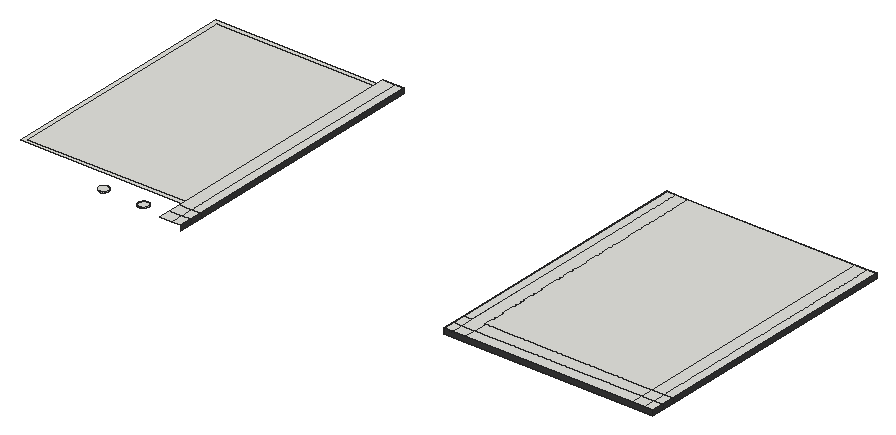
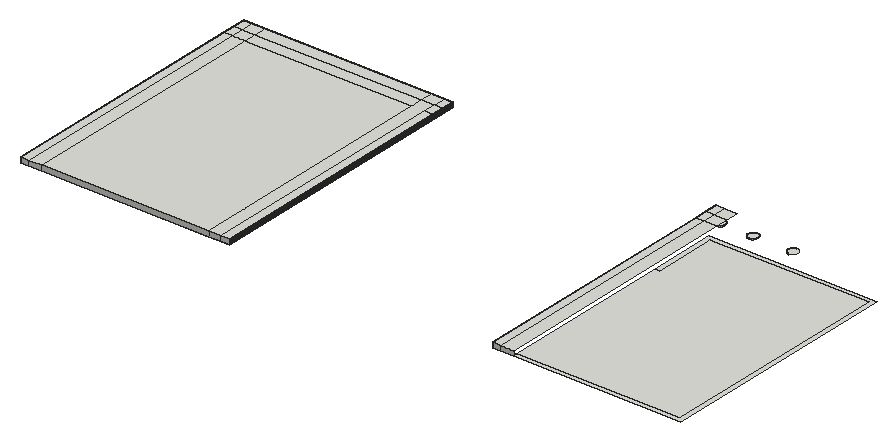
# SketchUp Ruby script. Lengths in inches.
U = 1.inch
M = Sketchup.active_model
def pt(a) = Geom::Point3d.new(a.map { |v| v * U })
def face(e, loops, mat)
  f = e.add_face(loops[0].map { |a| pt(a) })
  loops[1..].each { |l| e.add_face(l.map { |a| pt(a) }).erase! }
  f.material = f.back_material = mat if mat
  f
end
# faces: each face lists its corners as indices into pts; further lists are holes
def faces(e, pts, list, mat = nil) = list.each { |f| face(e, (f[0].is_a?(Array) ? f : [f]).map { |l| l.map { |i| pts[i] } }, mat) }
# xy, xz, yz: faces in a plane at the given z, y or x. An outline is a flat list of corners, or four numbers for a rectangle; further outlines are holes
def ring(l) = l.size == 4 ? [[l[0], l[1]], [l[2], l[1]], [l[2], l[3]], [l[0], l[3]]] : l.each_slice(2).to_a
def flat(e, list, mat, &to3) = list.each { |f| face(e, (f[0].is_a?(Array) ? f : [f]).map { |l| ring(l).map { |u, v| to3.(u, v) } }, mat) }
def xy(e, z, list, mat = nil) = flat(e, list, mat) { |x, y| [x, y, z] }
def xz(e, y, list, mat = nil) = flat(e, list, mat) { |x, z| [x, y, z] }
def yz(e, x, list, mat = nil) = flat(e, list, mat) { |y, z| [x, y, z] }
def lines(e, pts, list) = list.each { |a, b| e.add_line(pt(pts[a]), pt(pts[b])) }
# prism: a flat outline (further loops are holes) pulled along v
def prism(e, loops, v, mat = nil)
  f = face(e, loops, mat); d = Geom::Vector3d.new(v.map { |x| x * U })
  f.pushpull(f.normal.samedirection?(d) ? d.length : -d.length)
end
def box(e, o, s, mat = nil) = prism(e, [[o, [o[0] + s[0], o[1], o[2]], [o[0] + s[0], o[1] + s[1], o[2]], [o[0], o[1] + s[1], o[2]]]], [0, 0, s[2]], mat)
def at(x, y, z, deg = 0) = Geom::Transformation.translation(pt([x, y, z])) * Geom::Transformation.rotation(ORIGIN, Z_AXIS, deg.degrees)
def axes(o, x, y, z) = Geom::Transformation.new([*x, 0, *y, 0, *z, 0, *pt(o).to_a, 1])
def part(name) = M.definitions.add(name)
# library, detail: a bought-in or finely detailed component or shape, given as its bounding box
def library(name, o, s) = part(name).tap { |d| box(d.entities, o, s) }
def detail(e, o, s) = box(e.add_group.entities, o, s)
def put(e, d, t, mat = nil) = e.add_instance(d, t).tap { |i| i.material = mat if mat }
def group(e, t, mat = nil) = e.add_group.tap { |g| g.transformation = t; g.material = mat if mat }.entities
root = M.entities
M.materials.add("[Color C08]").color = [58, 29, 0]
M.materials.add("[Color M07]").color = [58, 58, 58]
xy(root,502.5625,[[649.1875,283.04,848.4,283.04,848.4,362.98,843.96,362.98,843.96,287.65,653.8,287.65,653.8,570.3125,848.4,570.3125,848.4,574.92,649.1875,574.92],[1212.3125,283.04,1411.53,283.04,1411.53,362.98,1407.08,362.98,1407.08,287.65,1216.92,287.65,1216.92,570.3125,1411.53,570.3125,1411.53,574.92,1212.3125,574.92],[653.8,287.65,653.8,570.3125,848.4,570.3125,848.4,362.98,843.96,362.98,843.96,287.65],[1216.92,287.65,1216.92,570.3125,1411.53,570.3125,1411.53,362.98,1407.08,362.98,1407.08,287.65],[848.4,570.3125,863.4,574.92],
  [863.4,570.3125,873.59,574.92],[1411.53,570.3125,1426.53,574.92],[1426.53,570.3125,1436.72,574.92]])
xy(root,502.5625,[[[1187.1875,241.85,1187.1875,574.92,1212.3125,574.92,1212.3125,283.04,1411.53,283.04,1411.53,570.3125,1436.72,570.3125,1436.72,241.85],[1332.08,251.93,1333.63,252.13,1335.08,252.72,1336.33,253.67,1337.29,254.91,1337.89,256.36,1338.1,257.91,1337.9,259.46,1337.3,260.91,1336.35,262.16,1335.11,263.12,1333.67,263.72,1332.12,263.93,1330.5625,263.73,1329.11,263.13,1327.87,262.18,1326.91,260.94,1326.31,259.5,1326.1,257.95,1326.3,256.39,1326.89,254.94,1327.84,253.7,1329.08,252.74,1330.53,252.14],[1213.89,251.93,1215.45,252.13,1216.9,252.72,1218.14,253.67,1219.1,254.91,1219.7,256.36,1219.91,257.91,1219.71,259.46,1219.12,260.91,1218.17,262.16,1216.93,263.12,1215.48,263.72,1213.93,263.93,1212.375,263.73,1210.93,263.13,1209.68,262.18,1208.72,260.94,1208.12,259.5,1207.91,257.95,1208.11,256.39,1208.71,254.94,1209.66,253.7,1210.9,252.74,1212.34,252.14],[1281.27,251.93,1282.82,252.13,1284.27,252.72,1285.52,253.67,1286.47,254.91,1287.08,256.36,1287.29,257.91,1287.09,259.46,1286.49,260.91,1285.54,262.16,1284.3,263.12,1282.86,263.72,1281.3,263.93,1279.75,263.73,1278.3,263.13,1277.06,262.18,1276.1,260.94,1275.5,259.5,1275.29,257.95,1275.49,256.39,1276.08,254.94,1277.03,253.7,1278.27,252.74,1279.72,252.14],[1379.33,251.93,1380.88,252.13,1382.33,252.72,1383.58,253.67,1384.54,254.91,1385.14,256.36,1385.35,257.91,1385.15,259.46,1384.55,260.91,1383.6,262.16,1382.36,263.12,1380.92,263.72,1379.37,263.93,1377.8125,263.73,1376.36,263.13,1375.12,262.18,1374.16,260.94,1373.56,259.5,1373.35,257.95,1373.55,256.39,1374.14,254.94,1375.09,253.7,1376.33,252.74,1377.78,252.14],[1418.71,251.93,1420.26,252.13,1421.71,252.72,1422.95,253.67,1423.91,254.91,1424.51,256.36,1424.72,257.91,1424.52,259.46,1423.93,260.91,1422.98,262.16,1421.74,263.12,1420.29,263.72,1418.74,263.93,1417.1875,263.73,1415.74,263.13,1414.49,262.18,1413.54,260.94,1412.93,259.5,1412.72,257.95,1412.92,256.39,1413.52,254.94,1414.47,253.7,1415.71,252.74,1417.15,252.14]]],"[Color C08]")
xy(root,503.4375,[[768.96,251.93,767.4,252.14,765.96,252.74,764.72,253.7,763.77,254.94,763.17,256.39,762.97,257.95,763.18,259.5,763.79,260.94,764.74,262.18,765.99,263.13,767.4375,263.73,768.99,263.93,770.54,263.72,771.99,263.12,773.23,262.16,774.18,260.91,774.77,259.46,774.97,257.91,774.76,256.36,774.16,254.91,773.2,253.67,771.96,252.72,770.51,252.13],[816.21,251.93,814.65,252.14,813.21,252.74,811.97,253.7,811.02,254.94,810.42,256.39,810.22,257.95,810.43,259.5,811.04,260.94,811.99,262.18,813.24,263.13,814.6875,263.73,816.24,263.93,817.79,263.72,819.24,263.12,820.48,262.16,821.43,260.91,822.02,259.46,822.22,257.91,822.01,256.36,821.41,254.91,820.45,253.67,819.21,252.72,817.76,252.13],[855.58,251.93,854.03,252.14,852.58,252.74,851.34,253.7,850.39,254.94,849.8,256.39,849.6,257.95,849.81,259.5,850.41,260.94,851.37,262.18,852.61,263.13,854.0625,263.73,855.62,263.93,857.17,263.72,858.61,263.12,859.85,262.16,860.8,260.91,861.4,259.46,861.6,257.91,861.39,256.36,860.79,254.91,859.83,253.67,858.58,252.72,857.13,252.13],[1213.89,251.93,1212.34,252.14,1210.9,252.74,1209.66,253.7,1208.71,254.94,1208.11,256.39,1207.91,257.95,1208.12,259.5,1208.72,260.94,1209.68,262.18,1210.93,263.13,1212.375,263.73,1213.93,263.93,1215.48,263.72,1216.93,263.12,1218.17,262.16,1219.12,260.91,1219.71,259.46,1219.91,257.91,1219.7,256.36,1219.1,254.91,1218.14,253.67,1216.9,252.72,1215.45,252.13],[1281.27,251.93,1279.72,252.14,1278.27,252.74,1277.03,253.7,1276.08,254.94,1275.49,256.39,1275.29,257.95,1275.5,259.5,1276.1,260.94,1277.06,262.18,1278.3,263.13,1279.75,263.73,1281.3,263.93,1282.86,263.72,1284.3,263.12,1285.54,262.16,1286.49,260.91,1287.09,259.46,1287.29,257.91,1287.08,256.36,1286.47,254.91,1285.52,253.67,1284.27,252.72,1282.82,252.13],
  [1332.08,251.93,1330.53,252.14,1329.08,252.74,1327.84,253.7,1326.89,254.94,1326.3,256.39,1326.1,257.95,1326.31,259.5,1326.91,260.94,1327.87,262.18,1329.11,263.13,1330.5625,263.73,1332.12,263.93,1333.67,263.72,1335.11,263.12,1336.35,262.16,1337.3,260.91,1337.9,259.46,1338.1,257.91,1337.89,256.36,1337.29,254.91,1336.33,253.67,1335.08,252.72,1333.63,252.13],[1379.33,251.93,1377.78,252.14,1376.33,252.74,1375.09,253.7,1374.14,254.94,1373.55,256.39,1373.35,257.95,1373.56,259.5,1374.16,260.94,1375.12,262.18,1376.36,263.13,1377.8125,263.73,1379.37,263.93,1380.92,263.72,1382.36,263.12,1383.6,262.16,1384.55,260.91,1385.15,259.46,1385.35,257.91,1385.14,256.36,1384.54,254.91,1383.58,253.67,1382.33,252.72,1380.88,252.13],[1418.71,251.93,1417.15,252.14,1415.71,252.74,1414.47,253.7,1413.52,254.94,1412.92,256.39,1412.72,257.95,1412.93,259.5,1413.54,260.94,1414.49,262.18,1415.74,263.13,1417.1875,263.73,1418.74,263.93,1420.29,263.72,1421.74,263.12,1422.98,262.16,1423.93,260.91,1424.52,259.46,1424.72,257.91,1424.51,256.36,1423.91,254.91,1422.95,253.67,1421.71,252.72,1420.26,252.13]])
xy(root,508.5625,[[848.4,241.85,863.4,256.29],[863.4,241.85,873.59,256.29],[1187.1875,241.85,1197.375,256.29],[1197.375,241.85,1212.3125,256.29],[1212.3125,241.85,1411.53,256.29],
  [1411.53,241.85,1426.53,256.29],[1426.53,241.85,1436.72,256.29],[848.4,256.29,863.4,271.23],[863.4,256.29,873.59,271.23],[1187.1875,256.29,1197.375,271.23],
  [1197.375,256.29,1212.3125,574.92],[1212.3125,256.29,1411.53,271.23],[1411.53,256.29,1426.53,271.23],[1426.53,256.29,1436.72,271.23],[848.4,271.23,863.4,574.92],
  [863.4,271.23,873.59,574.92],[1187.1875,271.23,1197.375,574.92],[1212.3125,271.23,1411.53,574.92],[1411.53,271.23,1426.53,574.92],[1426.53,271.23,1436.72,574.92]])
xz(root,241.85,[[1187.1875,502.5625,1436.72,508.5625]],"[Color M07]")
xz(root,574.92,[[848.4,502.5625,863.4,508.5625],[863.4,502.5625,873.59,508.5625],[1187.1875,502.5625,1197.375,508.5625],[1197.375,502.5625,1212.3125,508.5625],[1212.3125,502.5625,1411.53,508.5625],
  [1411.53,502.5625,1426.53,508.5625],[1426.53,502.5625,1436.72,508.5625]])
yz(root,873.59,[[241.85,502.5625,256.29,508.5625],[256.29,502.5625,271.23,508.5625],[271.23,502.5625,574.92,508.5625]],"[Color M07]")
yz(root,1187.1875,[[241.85,502.5625,256.29,508.5625],[256.29,502.5625,271.23,508.5625],[271.23,502.5625,574.92,508.5625]],"[Color M07]")
yz(root,1436.72,[[241.85,502.5625,256.29,508.5625],[256.29,502.5625,271.23,508.5625],[271.23,502.5625,574.92,508.5625]],"[Color M07]")
p = [[770.51,252.13,502.5625],[768.96,251.93,502.5625],[768.96,251.93,503.4375],[770.51,252.13,503.4375],[816.21,251.93,502.5625],[814.65,252.14,502.5625],
  [814.65,252.14,503.4375],[816.21,251.93,503.4375],[817.76,252.13,502.5625],[817.76,252.13,503.4375],[855.58,251.93,502.5625],[854.03,252.14,502.5625],
  [854.03,252.14,503.4375],[855.58,251.93,503.4375],[857.13,252.13,502.5625],[857.13,252.13,503.4375],[1213.89,251.93,502.5625],[1212.34,252.14,502.5625],
  [1212.34,252.14,503.4375],[1213.89,251.93,503.4375],[1215.45,252.13,502.5625],[1215.45,252.13,503.4375],[1281.27,251.93,502.5625],[1279.72,252.14,502.5625],
  [1279.72,252.14,503.4375],[1281.27,251.93,503.4375],[1282.82,252.13,502.5625],[1282.82,252.13,503.4375],[1332.08,251.93,502.5625],[1330.53,252.14,502.5625],
  [1330.53,252.14,503.4375],[1332.08,251.93,503.4375],[1333.63,252.13,502.5625],[1333.63,252.13,503.4375],[1379.33,251.93,502.5625],[1377.78,252.14,502.5625],
  [1377.78,252.14,503.4375],[1379.33,251.93,503.4375],[1380.88,252.13,502.5625],[1380.88,252.13,503.4375],[1418.71,251.93,502.5625],[1417.15,252.14,502.5625],
  [1417.15,252.14,503.4375],[1418.71,251.93,503.4375],[1420.26,252.13,502.5625],[1420.26,252.13,503.4375],[771.96,252.72,502.5625],[771.96,252.72,503.4375],
  [813.21,252.74,502.5625],[813.21,252.74,503.4375],[819.21,252.72,502.5625],[819.21,252.72,503.4375],[852.58,252.74,502.5625],[852.58,252.74,503.4375],
  [858.58,252.72,502.5625],[858.58,252.72,503.4375],[1210.9,252.74,502.5625],[1210.9,252.74,503.4375],[1216.9,252.72,502.5625],[1216.9,252.72,503.4375],
  [1278.27,252.74,502.5625],[1278.27,252.74,503.4375],[1284.27,252.72,502.5625],[1284.27,252.72,503.4375],[1329.08,252.74,502.5625],[1329.08,252.74,503.4375],
  [1335.08,252.72,502.5625],[1335.08,252.72,503.4375],[1376.33,252.74,502.5625],[1376.33,252.74,503.4375],[1382.33,252.72,502.5625],[1382.33,252.72,503.4375],
  [1415.71,252.74,502.5625],[1415.71,252.74,503.4375],[1421.71,252.72,502.5625],[1421.71,252.72,503.4375],[773.2,253.67,502.5625],[773.2,253.67,503.4375],
  [811.97,253.7,502.5625],[811.97,253.7,503.4375],[820.45,253.67,502.5625],[820.45,253.67,503.4375],[851.34,253.7,502.5625],[851.34,253.7,503.4375],
  [859.83,253.67,502.5625],[859.83,253.67,503.4375],[1209.66,253.7,502.5625],[1209.66,253.7,503.4375],[1218.14,253.67,502.5625],[1218.14,253.67,503.4375],
  [1277.03,253.7,502.5625],[1277.03,253.7,503.4375],[1285.52,253.67,502.5625],[1285.52,253.67,503.4375],[1327.84,253.7,502.5625],[1327.84,253.7,503.4375],
  [1336.33,253.67,502.5625],[1336.33,253.67,503.4375],[1375.09,253.7,502.5625],[1375.09,253.7,503.4375],[1383.58,253.67,502.5625],[1383.58,253.67,503.4375],
  [1414.47,253.7,502.5625],[1414.47,253.7,503.4375],[1422.95,253.67,502.5625],[1422.95,253.67,503.4375],[774.16,254.91,502.5625],[774.16,254.91,503.4375],
  [811.02,254.94,502.5625],[811.02,254.94,503.4375],[821.41,254.91,502.5625],[821.41,254.91,503.4375],[850.39,254.94,502.5625],[850.39,254.94,503.4375],
  [860.79,254.91,502.5625],[860.79,254.91,503.4375],[1208.71,254.94,502.5625],[1208.71,254.94,503.4375],[1219.1,254.91,502.5625],[1219.1,254.91,503.4375],
  [1276.08,254.94,502.5625],[1276.08,254.94,503.4375],[1286.47,254.91,502.5625],[1286.47,254.91,503.4375],[1326.89,254.94,502.5625],[1326.89,254.94,503.4375],
  [1337.29,254.91,502.5625],[1337.29,254.91,503.4375],[1374.14,254.94,502.5625],[1374.14,254.94,503.4375],[1384.54,254.91,502.5625],[1384.54,254.91,503.4375],
  [1413.52,254.94,502.5625],[1413.52,254.94,503.4375],[1423.91,254.91,502.5625],[1423.91,254.91,503.4375],[774.76,256.36,502.5625],[774.76,256.36,503.4375],
  [810.42,256.39,502.5625],[810.42,256.39,503.4375],[822.01,256.36,502.5625],[822.01,256.36,503.4375],[849.8,256.39,502.5625],[849.8,256.39,503.4375],
  [861.39,256.36,502.5625],[861.39,256.36,503.4375],[1208.11,256.39,502.5625],[1208.11,256.39,503.4375],[1219.7,256.36,502.5625],[1219.7,256.36,503.4375],
  [1275.49,256.39,502.5625],[1275.49,256.39,503.4375],[1287.08,256.36,502.5625],[1287.08,256.36,503.4375],[1326.3,256.39,502.5625],[1326.3,256.39,503.4375],
  [1337.89,256.36,502.5625],[1337.89,256.36,503.4375],[1373.55,256.39,502.5625],[1373.55,256.39,503.4375],[1385.14,256.36,502.5625],[1385.14,256.36,503.4375],
  [1412.92,256.39,502.5625],[1412.92,256.39,503.4375],[1424.51,256.36,502.5625],[1424.51,256.36,503.4375],[774.97,257.91,502.5625],[774.97,257.91,503.4375],
  [810.22,257.95,502.5625],[810.22,257.95,503.4375],[822.22,257.91,502.5625],[822.22,257.91,503.4375],[849.6,257.95,502.5625],[849.6,257.95,503.4375],
  [861.6,257.91,502.5625],[861.6,257.91,503.4375],[1207.91,257.95,502.5625],[1207.91,257.95,503.4375],[1219.91,257.91,502.5625],[1219.91,257.91,503.4375],
  [1275.29,257.95,502.5625],[1275.29,257.95,503.4375],[1287.29,257.91,502.5625],[1287.29,257.91,503.4375],[1326.1,257.95,502.5625],[1326.1,257.95,503.4375],
  [1338.1,257.91,502.5625],[1338.1,257.91,503.4375],[1373.35,257.95,502.5625],[1373.35,257.95,503.4375],[1385.35,257.91,502.5625],[1385.35,257.91,503.4375],
  [1412.72,257.95,502.5625],[1412.72,257.95,503.4375],[1424.72,257.91,502.5625],[1424.72,257.91,503.4375],[774.77,259.46,502.5625],[774.77,259.46,503.4375],
  [810.43,259.5,502.5625],[810.43,259.5,503.4375],[822.02,259.46,502.5625],[822.02,259.46,503.4375],[849.81,259.5,502.5625],[849.81,259.5,503.4375],
  [861.4,259.46,502.5625],[861.4,259.46,503.4375],[1208.12,259.5,502.5625],[1208.12,259.5,503.4375],[1219.71,259.46,502.5625],[1219.71,259.46,503.4375],
  [1275.5,259.5,502.5625],[1275.5,259.5,503.4375],[1287.09,259.46,502.5625],[1287.09,259.46,503.4375],[1326.31,259.5,502.5625],[1326.31,259.5,503.4375],
  [1337.9,259.46,502.5625],[1337.9,259.46,503.4375],[1373.56,259.5,502.5625],[1373.56,259.5,503.4375],[1385.15,259.46,502.5625],[1385.15,259.46,503.4375],
  [1412.93,259.5,502.5625],[1412.93,259.5,503.4375],[1424.52,259.46,502.5625],[1424.52,259.46,503.4375],[774.18,260.91,502.5625],[774.18,260.91,503.4375],
  [811.04,260.94,502.5625],[811.04,260.94,503.4375],[821.43,260.91,502.5625],[821.43,260.91,503.4375],[850.41,260.94,502.5625],[850.41,260.94,503.4375],
  [860.8,260.91,502.5625],[860.8,260.91,503.4375],[1208.72,260.94,502.5625],[1208.72,260.94,503.4375],[1219.12,260.91,502.5625],[1219.12,260.91,503.4375],
  [1276.1,260.94,502.5625],[1276.1,260.94,503.4375],[1286.49,260.91,502.5625],[1286.49,260.91,503.4375],[1326.91,260.94,502.5625],[1326.91,260.94,503.4375],
  [1337.3,260.91,502.5625],[1337.3,260.91,503.4375],[1374.16,260.94,502.5625],[1374.16,260.94,503.4375],[1384.55,260.91,502.5625],[1384.55,260.91,503.4375],
  [1413.54,260.94,502.5625],[1413.54,260.94,503.4375],[1423.93,260.91,502.5625],[1423.93,260.91,503.4375],[773.23,262.16,502.5625],[773.23,262.16,503.4375],
  [811.99,262.18,502.5625],[811.99,262.18,503.4375],[820.48,262.16,502.5625],[820.48,262.16,503.4375],[851.37,262.18,502.5625],[851.37,262.18,503.4375],
  [859.85,262.16,502.5625],[859.85,262.16,503.4375],[1209.68,262.18,502.5625],[1209.68,262.18,503.4375],[1218.17,262.16,502.5625],[1218.17,262.16,503.4375],
  [1277.06,262.18,502.5625],[1277.06,262.18,503.4375],[1285.54,262.16,502.5625],[1285.54,262.16,503.4375],[1327.87,262.18,502.5625],[1327.87,262.18,503.4375],
  [1336.35,262.16,502.5625],[1336.35,262.16,503.4375],[1375.12,262.18,502.5625],[1375.12,262.18,503.4375],[1383.6,262.16,502.5625],[1383.6,262.16,503.4375],
  [1414.49,262.18,502.5625],[1414.49,262.18,503.4375],[1422.98,262.16,502.5625],[1422.98,262.16,503.4375],[771.99,263.12,502.5625],[771.99,263.12,503.4375],
  [813.24,263.13,502.5625],[813.24,263.13,503.4375],[819.24,263.12,502.5625],[819.24,263.12,503.4375],[852.61,263.13,502.5625],[852.61,263.13,503.4375],
  [858.61,263.12,502.5625],[858.61,263.12,503.4375],[1210.93,263.13,502.5625],[1210.93,263.13,503.4375],[1216.93,263.12,502.5625],[1216.93,263.12,503.4375],
  [1278.3,263.13,502.5625],[1278.3,263.13,503.4375],[1284.3,263.12,502.5625],[1284.3,263.12,503.4375],[1329.11,263.13,502.5625],[1329.11,263.13,503.4375],
  [1335.11,263.12,502.5625],[1335.11,263.12,503.4375],[1376.36,263.13,502.5625],[1376.36,263.13,503.4375],[1382.36,263.12,502.5625],[1382.36,263.12,503.4375],
  [1415.74,263.13,502.5625],[1415.74,263.13,503.4375],[1421.74,263.12,502.5625],[1421.74,263.12,503.4375],[770.54,263.72,502.5625],[770.54,263.72,503.4375],
  [814.6875,263.73,502.5625],[814.6875,263.73,503.4375],[817.79,263.72,502.5625],[817.79,263.72,503.4375],[854.0625,263.73,502.5625],[854.0625,263.73,503.4375],
  [857.17,263.72,502.5625],[857.17,263.72,503.4375],[1212.375,263.73,502.5625],[1212.375,263.73,503.4375],[1215.48,263.72,502.5625],[1215.48,263.72,503.4375],
  [1279.75,263.73,502.5625],[1279.75,263.73,503.4375],[1282.86,263.72,502.5625],[1282.86,263.72,503.4375],[1330.5625,263.73,502.5625],[1330.5625,263.73,503.4375],
  [1333.67,263.72,502.5625],[1333.67,263.72,503.4375],[1377.8125,263.73,502.5625],[1377.8125,263.73,503.4375],[1380.92,263.72,502.5625],[1380.92,263.72,503.4375],
  [1417.1875,263.73,502.5625],[1417.1875,263.73,503.4375],[1420.29,263.72,502.5625],[1420.29,263.72,503.4375],[768.99,263.93,502.5625],[768.99,263.93,503.4375],
  [816.24,263.93,502.5625],[816.24,263.93,503.4375],[855.62,263.93,502.5625],[855.62,263.93,503.4375],[1213.93,263.93,502.5625],[1213.93,263.93,503.4375],
  [1281.3,263.93,502.5625],[1281.3,263.93,503.4375],[1332.12,263.93,502.5625],[1332.12,263.93,503.4375],[1379.37,263.93,502.5625],[1379.37,263.93,503.4375],
  [1418.74,263.93,502.5625],[1418.74,263.93,503.4375],[1197.375,256.29,502.5625],[1197.375,256.29,508.5625],[1212.3125,256.29,502.5625],[1212.3125,256.29,508.5625]]
faces(root,p,[[0,1,2,3],[4,5,6,7],[8,4,7,9],[10,11,12,13],[14,10,13,15],[16,17,18,19],[20,16,19,21],[22,23,24,25],
  [26,22,25,27],[28,29,30,31],[32,28,31,33],[34,35,36,37],[38,34,37,39],[40,41,42,43],[44,40,43,45],[46,0,3,47],
  [5,48,49,6],[50,8,9,51],[11,52,53,12],[54,14,15,55],[17,56,57,18],[58,20,21,59],[23,60,61,24],[62,26,27,63],
  [29,64,65,30],[66,32,33,67],[35,68,69,36],[70,38,39,71],[41,72,73,42],[74,44,45,75],[76,46,47,77],[48,78,79,49],
  [80,50,51,81],[52,82,83,53],[84,54,55,85],[56,86,87,57],[88,58,59,89],[60,90,91,61],[92,62,63,93],[64,94,95,65],
  [96,66,67,97],[68,98,99,69],[100,70,71,101],[72,102,103,73],[104,74,75,105],[106,76,77,107],[78,108,109,79],[110,80,81,111],
  [82,112,113,83],[114,84,85,115],[86,116,117,87],[118,88,89,119],[90,120,121,91],[122,92,93,123],[94,124,125,95],[126,96,97,127],
  [98,128,129,99],[130,100,101,131],[102,132,133,103],[134,104,105,135],[136,106,107,137],[108,138,139,109],[140,110,111,141],[112,142,143,113],
  [144,114,115,145],[116,146,147,117],[148,118,119,149],[120,150,151,121],[152,122,123,153],[124,154,155,125],[156,126,127,157],[128,158,159,129],
  [160,130,131,161],[132,162,163,133],[164,134,135,165],[166,136,137,167],[138,168,169,139],[170,140,141,171],[142,172,173,143],[174,144,145,175],
  [146,176,177,147],[178,148,149,179],[150,180,181,151],[182,152,153,183],[154,184,185,155],[186,156,157,187],[158,188,189,159],[190,160,161,191],
  [162,192,193,163],[194,164,165,195],[196,166,167,197],[168,198,199,169],[200,170,171,201],[172,202,203,173],[204,174,175,205],[176,206,207,177],
  [208,178,179,209],[180,210,211,181],[212,182,183,213],[184,214,215,185],[216,186,187,217],[188,218,219,189],[220,190,191,221],[192,222,223,193],
  [224,194,195,225],[226,196,197,227],[198,228,229,199],[230,200,201,231],[202,232,233,203],[234,204,205,235],[206,236,237,207],[238,208,209,239],
  [210,240,241,211],[242,212,213,243],[214,244,245,215],[246,216,217,247],[218,248,249,219],[250,220,221,251],[222,252,253,223],[254,224,225,255],
  [256,226,227,257],[228,258,259,229],[260,230,231,261],[232,262,263,233],[264,234,235,265],[236,266,267,237],[268,238,239,269],[240,270,271,241],
  [272,242,243,273],[244,274,275,245],[276,246,247,277],[248,278,279,249],[280,250,251,281],[252,282,283,253],[284,254,255,285],[286,256,257,287],
  [258,288,289,259],[290,260,261,291],[262,292,293,263],[294,264,265,295],[266,296,297,267],[298,268,269,299],[270,300,301,271],[302,272,273,303],
  [274,304,305,275],[306,276,277,307],[278,308,309,279],[310,280,281,311],[282,312,313,283],[314,284,285,315],[316,286,287,317],[288,318,319,289],
  [320,290,291,321],[292,322,323,293],[324,294,295,325],[296,326,327,297],[328,298,299,329],[300,330,331,301],[332,302,303,333],[304,334,335,305],
  [336,306,307,337],[308,338,339,309],[340,310,311,341],[312,342,343,313],[344,314,315,345],[346,316,317,347],[318,348,349,319],[348,320,321,349],
  [322,350,351,323],[350,324,325,351],[326,352,353,327],[352,328,329,353],[330,354,355,331],[354,332,333,355],[334,356,357,335],[356,336,337,357],
  [338,358,359,339],[358,340,341,359],[342,360,361,343],[360,344,345,361]])
lines(root,p,[[362,363],[364,365]])
